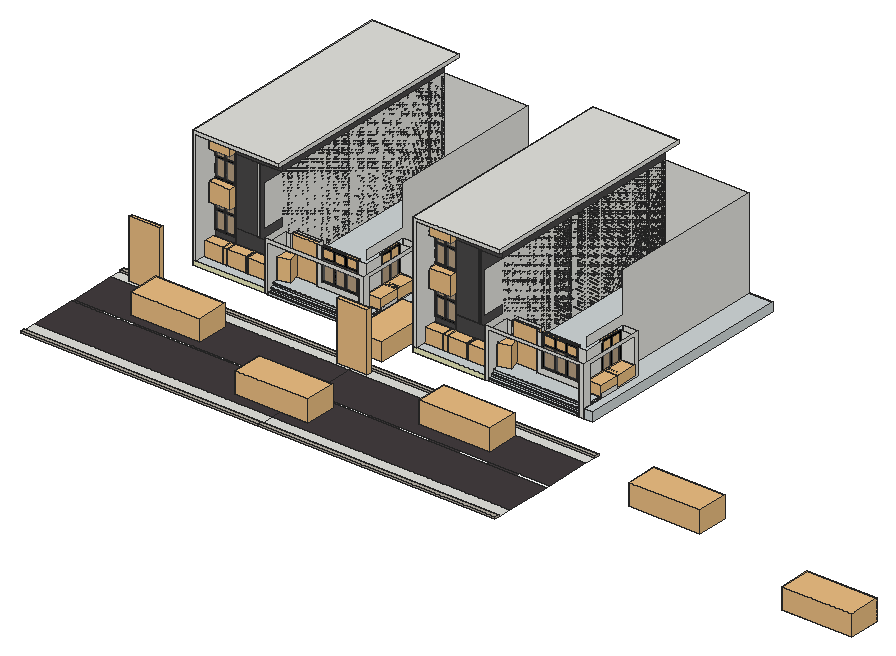
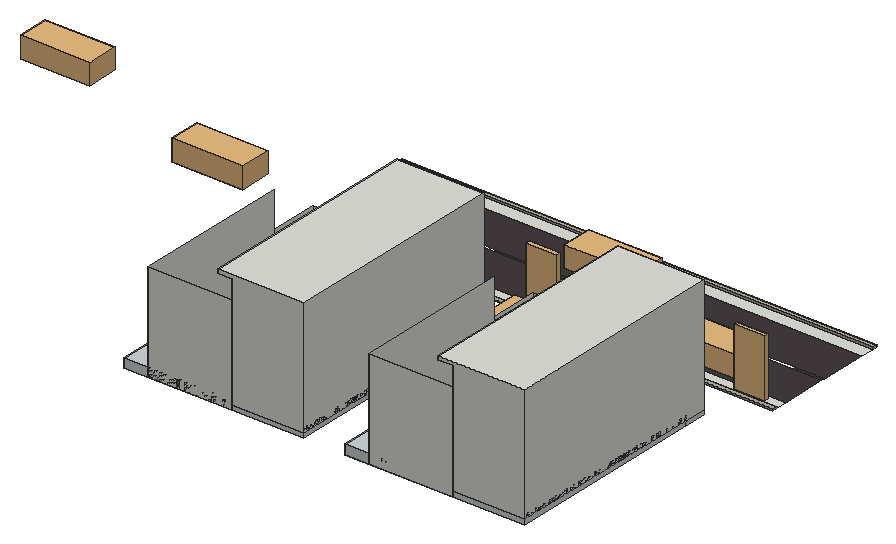
# SketchUp Ruby script. Lengths in inches.
U = 1.inch
M = Sketchup.active_model
def pt(a) = Geom::Point3d.new(a.map { |v| v * U })
def face(e, loops, mat)
  f = e.add_face(loops[0].map { |a| pt(a) })
  loops[1..].each { |l| e.add_face(l.map { |a| pt(a) }).erase! }
  f.material = f.back_material = mat if mat
  f
end
# faces: each face lists its corners as indices into pts; further lists are holes
def faces(e, pts, list, mat = nil) = list.each { |f| face(e, (f[0].is_a?(Array) ? f : [f]).map { |l| l.map { |i| pts[i] } }, mat) }
# xy, xz, yz: faces in a plane at the given z, y or x. An outline is a flat list of corners, or four numbers for a rectangle; further outlines are holes
def ring(l) = l.size == 4 ? [[l[0], l[1]], [l[2], l[1]], [l[2], l[3]], [l[0], l[3]]] : l.each_slice(2).to_a
def flat(e, list, mat, &to3) = list.each { |f| face(e, (f[0].is_a?(Array) ? f : [f]).map { |l| ring(l).map { |u, v| to3.(u, v) } }, mat) }
def xy(e, z, list, mat = nil) = flat(e, list, mat) { |x, y| [x, y, z] }
def xz(e, y, list, mat = nil) = flat(e, list, mat) { |x, z| [x, y, z] }
def yz(e, x, list, mat = nil) = flat(e, list, mat) { |y, z| [x, y, z] }
def lines(e, pts, list) = list.each { |a, b| e.add_line(pt(pts[a]), pt(pts[b])) }
# prism: a flat outline (further loops are holes) pulled along v
def prism(e, loops, v, mat = nil)
  f = face(e, loops, mat); d = Geom::Vector3d.new(v.map { |x| x * U })
  f.pushpull(f.normal.samedirection?(d) ? d.length : -d.length)
end
def box(e, o, s, mat = nil) = prism(e, [[o, [o[0] + s[0], o[1], o[2]], [o[0] + s[0], o[1] + s[1], o[2]], [o[0], o[1] + s[1], o[2]]]], [0, 0, s[2]], mat)
def at(x, y, z, deg = 0) = Geom::Transformation.translation(pt([x, y, z])) * Geom::Transformation.rotation(ORIGIN, Z_AXIS, deg.degrees)
def axes(o, x, y, z) = Geom::Transformation.new([*x, 0, *y, 0, *z, 0, *pt(o).to_a, 1])
def part(name) = M.definitions.add(name)
# library, detail: a bought-in or finely detailed component or shape, given as its bounding box
def library(name, o, s) = part(name).tap { |d| box(d.entities, o, s) }
def detail(e, o, s) = box(e.add_group.entities, o, s)
def put(e, d, t, mat = nil) = e.add_instance(d, t).tap { |i| i.material = mat if mat }
def group(e, t, mat = nil) = e.add_group.tap { |g| g.transformation = t; g.material = mat if mat }.entities
root = M.entities
M.materials.add("1408 AP K082 Hot Ganache-N").color = [74, 72, 72]
M.materials.add("Polycor-Pavers-GEORGIA-MARBLEtm-PEARL-GREY-Tranche-1-4K").color = [207, 214, 215]
M.materials.add("Teddy_Paper").color = [237, 237, 189]
M.materials.add("[Asphalt_New]").color = [67, 60, 62]
M.materials.add("[Color A05]").color = [255, 0, 0]
M.materials.add("[Color M09]").color = [0, 0, 0]
M.materials.add("[Color_000]").color = [255, 255, 255]
M.materials.add("[Stone_Masonry_Multi]").color = [182, 175, 164]
M.materials.add("[Translucent Glass Gray]").color = [128, 128, 128]
M.materials["[Translucent Glass Gray]"].alpha = 0.5
c1 = library("Street Lighting Pole",[31.3125,-4.22,0],[127.34,10.44,259.08])
c2 = library("Group13",[-203.48,36.63,0],[29.68,67.31,50.64])
c3 = library("Group13\#2",[-203.48,36.63,0],[29.68,67.31,50.64])
c4 = part("Group\#61")
p = [[0,1.89,0.38],[0,1.89,1.61],[0,0.72,0],[0,0,0.99],[0,0.72,1.99]]
lines(c4.entities,p,[[0,1],[2,0],[3,2],[4,3],[1,4]])
c5 = part("Component\#76")
p = [[20.45,2.26,80],[20.78,2.41,80]]
lines(c5.entities,p,[[0,1]])
detail(c5.entities,[0,1.93,2.7],[20.05,3.87,77.3])
put(c5.entities,c4,at(9.77,5.02,80,-180))
put(c5.entities,c4,at(11.91,5.02,80,-180))
put(c5.entities,c4,at(13.54,5.02,80,-180))
put(c5.entities,c4,at(7.29,5.02,80,-180))
put(c5.entities,c4,at(6.18,5.02,80,-180))
put(c5.entities,c4,at(8.69,5.02,80,-180))
put(c5.entities,c4,at(17.42,5.04,80,-180))
put(c5.entities,c4,at(18.86,5.04,80,-180))
put(c5.entities,c4,at(15.09,5.02,80,-180))
put(c5.entities,c4,at(16.66,5.04,80,-180))
put(c5.entities,c4,at(2.54,5.02,80,-180))
put(c5.entities,c4,at(1.38,5.02,80,-180))
put(c5.entities,c4,at(4.1,5.02,80,-180))
c6 = library("Group96\#1",[-28.47,-25.5,0],[56.94,51,19.8125])
c7 = library("Group112\#2",[-28.47,-24.66,0],[56.94,49.32,19.8125])
c8 = library("cay+chuoi",[36.12,19.66,0.52],[32.73,35.6,54.38])
c9 = part("weg 1")
xy(c9.entities,0,[[119.79,-0.03,149.12,635.01],[405.36,-0.03,441.44,635.01]])
xy(c9.entities,0,[[149.12,-0.03,272.68,635.01],[272.68,-0.03,280.61,79.35],[280.61,-0.03,405.36,635.01],[272.68,158.73,280.61,238.11],[272.68,317.49,280.61,396.87],
  [272.68,476.25,280.61,555.63]],"[Asphalt_New]")
xy(c9.entities,0,[[272.68,79.35,280.61,158.73],[272.68,238.11,280.61,317.49],[272.68,396.87,280.61,476.25],[272.68,555.63,280.61,635.01]],"[Color_000]")
xy(c9.entities,4.33,[[108.17,0,119.79,635.01]],"[Stone_Masonry_Multi]")
xy(c9.entities,5.12,[[441.44,-0.03,453.25,635.01]],"[Stone_Masonry_Multi]")
xz(c9.entities,-0.03,[[441.44,0,453.25,5.12]],"[Stone_Masonry_Multi]")
xz(c9.entities,0,[[108.17,0,119.79,4.33]],"[Stone_Masonry_Multi]")
xz(c9.entities,635.01,[[108.17,0,119.79,4.33],[441.44,0,453.25,5.12]],"[Stone_Masonry_Multi]")
yz(c9.entities,108.17,[[0,0,635.01,4.33]],"[Stone_Masonry_Multi]")
yz(c9.entities,119.79,[[0,0,635.01,4.33]],"[Stone_Masonry_Multi]")
yz(c9.entities,441.44,[[-0.03,0,635.01,5.12]],"[Stone_Masonry_Multi]")
yz(c9.entities,453.25,[[-0.03,0,635.01,5.12]],"[Stone_Masonry_Multi]")
c10 = part("Group\#1")
xy(c10.entities,-18,[[0,0,192,60],[456.375,0,456.375,60,449.99,60,449.99,7.5,442.99,7.5,442.99,1,200.82,1,200.82,60,0,60,0,600,480,600,480,0]])
xy(c10.entities,-12.875,[[7.5,33,184.5,52.5]])
xy(c10.entities,-12,[[200.82,0,442.99,1]])
xy(c10.entities,-10,[[200.82,0,442.99,8.5]],"Polycor-Pavers-GEORGIA-MARBLEtm-PEARL-GREY-Tranche-1-4K")
xy(c10.entities,-5.0625,[[[0,0,192,60],[7.5,33,184.5,52.5]]])
xy(c10.entities,-4,[[200.82,7.5,442.99,8.5]])
xy(c10.entities,-2,[[200.82,7.5,442.99,16]],"Polycor-Pavers-GEORGIA-MARBLEtm-PEARL-GREY-Tranche-1-4K")
xy(c10.entities,4,[[200.82,15,442.99,16]])
xy(c10.entities,6,[[456.375,0,480,0,480,600,0,600,0,60,200.82,60,200.82,15,442.99,15,442.99,7.5,449.99,7.5,449.99,60,456.375,60]],"Polycor-Pavers-GEORGIA-MARBLEtm-PEARL-GREY-Tranche-1-4K")
xz(c10.entities,0,[[456.375,-18,480,6]])
xz(c10.entities,0,[[200.82,-12,442.99,-10]],"Polycor-Pavers-GEORGIA-MARBLEtm-PEARL-GREY-Tranche-1-4K")
xz(c10.entities,0,[[0,-18,192,-5.0625]],"Teddy_Paper")
xz(c10.entities,1,[[200.82,-18,442.99,-12]],"Polycor-Pavers-GEORGIA-MARBLEtm-PEARL-GREY-Tranche-1-4K")
xz(c10.entities,7.5,[[442.99,-18,449.99,6]])
xz(c10.entities,7.5,[[200.82,-4,442.99,-2]],"Polycor-Pavers-GEORGIA-MARBLEtm-PEARL-GREY-Tranche-1-4K")
xz(c10.entities,8.5,[[200.82,-10,442.99,-4]],"Polycor-Pavers-GEORGIA-MARBLEtm-PEARL-GREY-Tranche-1-4K")
xz(c10.entities,15,[[200.82,4,442.99,6]],"Polycor-Pavers-GEORGIA-MARBLEtm-PEARL-GREY-Tranche-1-4K")
xz(c10.entities,16,[[200.82,-2,442.99,4]],"Polycor-Pavers-GEORGIA-MARBLEtm-PEARL-GREY-Tranche-1-4K")
xz(c10.entities,33,[[7.5,-12.875,184.5,-5.0625]])
xz(c10.entities,52.5,[[7.5,-12.875,184.5,-5.0625]])
xz(c10.entities,60,[[0,-18,192,-5.0625],[192,-18,200.82,6],[449.99,-18,456.375,6],[0,-5.0625,192,6]])
xz(c10.entities,600,[[0,-18,480,6]])
yz(c10.entities,0,[[0,-18,60,-5.0625],[60,-18,600,6]])
yz(c10.entities,7.5,[[33,-12.875,52.5,-5.0625]])
yz(c10.entities,184.5,[[33,-12.875,52.5,-5.0625]])
yz(c10.entities,192,[[0,-18,60,-5.0625]])
yz(c10.entities,200.82,[[1,-18,1,-12,0,-12,0,-10,8.5,-10,8.5,-4,7.5,-4,7.5,-2,16,-2,16,4,15,4,15,6,60,6,60,-18]])
yz(c10.entities,442.99,[[1,-18,7.5,-18,7.5,-10,0,-10,0,-12,1,-12],[7.5,-10,8.5,-4],[7.5,-2,7.5,6,15,6,15,4,16,4,16,-2]])
yz(c10.entities,449.99,[[7.5,-18,60,6]])
yz(c10.entities,456.375,[[0,-18,60,6]])
yz(c10.entities,480,[[0,-18,600,6]])
c11 = library("Component",[-22.57,36.53,5.61],[7.19,69.19,99.57])
c12 = library("curtain",[-132.09,64.9,20.5],[94.35,4.27,84.68])
c13 = library("Group8",[-183.25,9.15,0],[25.91,56.79,43.93])
c14 = library("Untitled\#1",[-3930.05,580.88,0.02],[81.53,169.31,48.44])
c15 = library("bmw m6",[0,0,0],[74.56,175.18,49.66])
c16 = library("araç",[-7.9,-14.14,0],[84.07,190.26,56.29])
c17 = library("MERCEDES LIGHT",[-74.97,-97.73,0.18],[82.22,195.9,56.22])
c18 = part("cars")
put(c18.entities,c15,axes([-854.13,88.1875,0],[0,1.12,0],[-1.05539,0,0],[0,0,1.12246]))
put(c18.entities,c16,at(-104.32,108.73,0,90))
put(c18.entities,c17,at(-555.31,27.51,5.12,90))
put(c18.entities,c16,at(456.62,108.73,0,90))
put(c18.entities,c15,axes([807.37,-43.625,0],[0,1.12,0],[1.05539,0,0],[0,0,1.12246]))
xy(root,-4.3125,[[293.22,449.7,293.22,1049.7,518.04,1049.7,518.04,629.7,557.59,629.7,557.59,449.7,551.21,449.7,551.21,509.7,384.73,509.7,384.73,530.01,315.54,530.01,315.54,509.7,302.04,509.7,302.04,449.7],[544.21,449.7,551.21,457.2],[883.03,449.7,883.03,1049.7,1107.85,1049.7,1107.85,629.7,1147.4,629.7,1147.4,449.7,1141.02,449.7,1141.02,509.7,974.54,509.7,974.54,530.01,905.35,530.01,905.35,509.7,891.85,509.7,891.85,449.7],[1134.02,449.7,1141.02,457.2]])
xy(root,19.6875,[[551.21,468.65,557.59,509.7],[1141.02,468.65,1147.4,509.7]])
xy(root,22.13,[[522.83,514.49,552.8,616.09],[1112.64,514.49,1142.62,616.09]])
xy(root,28.51,[[[518.04,509.7,557.59,620.88],[522.83,514.49,552.8,616.09]],[[1107.85,509.7,1147.4,620.88],[1112.64,514.49,1142.62,616.09]]])
xy(root,34.1875,[[398.04,512.7,430.93,533.7],[430.93,512.7,461.15,533.7],[461.15,512.7,494.04,533.7],[987.85,512.7,1020.74,533.7],[1020.74,512.7,1050.96,533.7],
  [1050.96,512.7,1083.85,533.7]])
xy(root,34.1875,[[398.04,509.7,494.04,512.7],[987.85,509.7,1083.85,512.7],[516.04,559.44,518.04,590.16],[1105.85,559.44,1107.85,590.16],[516.04,590.16,518.04,620.88],
  [1105.85,590.16,1107.85,620.88]],"[Color M09]")
xy(root,34.86,[[501.6,560.12,516.04,591.16],[1091.41,560.12,1105.85,591.16],[501.6,591.16,516.04,620.2],[1091.41,591.16,1105.85,620.2]])
xy(root,36.86,[[400.71,509.7,430.93,511.2],[433.56,509.7,461.15,511.2],[463.98,509.7,491.36,511.2],[990.53,509.7,1020.74,511.2],[1023.37,509.7,1050.96,511.2],
  [1053.79,509.7,1081.17,511.2],[400.71,511.2,430.93,512.7],[433.56,511.2,461.15,512.7],[463.98,511.2,491.36,512.7],[990.53,511.2,1020.74,512.7],
  [1023.37,511.2,1050.96,512.7],[1053.79,511.2,1081.17,512.7],[516.04,562.12,517.04,589.16],[517.04,562.12,518.04,589.16],[1105.85,562.12,1106.85,589.16],
  [1106.85,562.12,1107.85,589.16],[516.04,589.16,518.04,590.16],[1105.85,589.16,1107.85,590.16],[516.04,590.16,518.04,591.16],[1105.85,590.16,1107.85,591.16],
  [516.04,591.16,517.04,618.2],[517.04,591.16,518.04,618.2],[1105.85,591.16,1106.85,618.2],[1106.85,591.16,1107.85,618.2]],"[Color M09]")
xz(root,449.7,[[293.22,-4.3125,302.04,-4.3125,302.04,118.87,544.21,118.87,544.21,-4.3125,557.59,-4.3125,557.59,127.6875,293.22,127.6875],[883.03,-4.3125,891.85,-4.3125,891.85,118.87,1134.02,118.87,1134.02,-4.3125,1147.4,-4.3125,1147.4,127.6875,883.03,127.6875]])
xz(root,457.2,[[544.21,-4.3125,551.21,118.87],[1134.02,-4.3125,1141.02,118.87]])
xz(root,468.65,[[551.21,19.6875,557.59,118.87],[1141.02,19.6875,1147.4,118.87]])
xz(root,509.7,[[302.04,-4.3125,315.54,118.87],[384.73,-4.3125,551.21,-4.3125,551.21,28.51,518.04,28.51,518.04,118.87,494.04,118.87,494.04,34.1875,398.04,34.1875,398.04,118.87,384.73,118.87],[891.85,-4.3125,905.35,118.87],[974.54,-4.3125,1141.02,-4.3125,1141.02,28.51,1107.85,28.51,1107.85,118.87,1083.85,118.87,1083.85,34.1875,987.85,34.1875,987.85,118.87,974.54,118.87],[551.21,19.6875,557.59,28.51],
  [1141.02,19.6875,1147.4,28.51]])
xz(root,509.7,[[[398.04,34.1875,494.04,118.87],[400.71,36.86,430.93,89.9],[433.56,36.86,461.15,89.9],[463.98,36.86,491.36,89.9],[400.71,92.58,430.93,116.1875],[433.56,92.58,461.15,116.1875],[463.98,92.58,491.36,116.1875]],[[987.85,34.1875,1083.85,118.87],[990.53,36.86,1020.74,89.9],[1023.37,36.86,1050.96,89.9],[1053.79,36.86,1081.17,89.9],[990.53,92.58,1020.74,116.1875],[1023.37,92.58,1050.96,116.1875],[1053.79,92.58,1081.17,116.1875]]],"[Color M09]")
xz(root,511.2,[[400.71,36.86,430.93,89.9],[433.56,36.86,461.15,89.9],[463.98,36.86,491.36,89.9],[990.53,36.86,1020.74,89.9],[1023.37,36.86,1050.96,89.9],
  [1053.79,36.86,1081.17,89.9]],"[Translucent Glass Gray]")
xz(root,512.7,[[430.93,34.1875,433.56,89.9],[1020.74,34.1875,1023.37,89.9]])
xz(root,512.7,[[398.04,34.1875,430.93,36.86],[433.56,34.1875,461.15,36.86],[461.15,34.1875,463.98,89.9],[463.98,34.1875,491.36,36.86],[491.36,34.1875,494.04,89.9],
  [987.85,34.1875,1020.74,36.86],[1023.37,34.1875,1050.96,36.86],[1050.96,34.1875,1053.79,89.9],[1053.79,34.1875,1081.17,36.86],[1081.17,34.1875,1083.85,89.9],
  [398.04,36.86,400.71,89.9],[987.85,36.86,990.53,89.9]],"[Color M09]")
xz(root,514.49,[[522.83,22.13,551.21,28.51],[551.21,22.13,552.8,28.51],[1112.64,22.13,1141.02,28.51],[1141.02,22.13,1142.62,28.51]])
xz(root,530.01,[[315.54,-4.3125,384.73,118.87],[905.35,-4.3125,974.54,118.87]])
xz(root,533.7,[[398.04,34.1875,430.93,89.9],[430.93,34.1875,461.15,89.9],[461.15,34.1875,494.04,89.9],[987.85,34.1875,1020.74,89.9],[1020.74,34.1875,1050.96,89.9],
  [1050.96,34.1875,1083.85,89.9]])
xz(root,559.44,[[516.04,34.1875,518.04,118.87],[1105.85,34.1875,1107.85,118.87]],"[Color M09]")
xz(root,560.12,[[501.6,34.86,516.04,89.9],[1091.41,34.86,1105.85,89.9]])
xz(root,561.12,[[516.04,36.86,518.04,89.9],[1105.85,36.86,1107.85,89.9]])
xz(root,562.12,[[516.04,36.86,517.04,89.9],[517.04,36.86,518.04,89.9],[1105.85,36.86,1106.85,89.9],[1106.85,36.86,1107.85,89.9]],"[Color M09]")
xz(root,589.16,[[516.04,36.86,517.04,89.9],[517.04,36.86,518.04,89.9],[1105.85,36.86,1106.85,89.9],[1106.85,36.86,1107.85,89.9]],"[Color M09]")
xz(root,590.16,[[516.04,34.1875,518.04,36.86],[1105.85,34.1875,1107.85,36.86]],"[Color M09]")
xz(root,591.16,[[516.04,36.86,517.04,89.9],[517.04,36.86,518.04,89.9],[1105.85,36.86,1106.85,89.9],[1106.85,36.86,1107.85,89.9]],"[Color M09]")
xz(root,616.09,[[522.83,22.13,552.8,28.51],[1112.64,22.13,1142.62,28.51]])
xz(root,618.2,[[516.04,36.86,517.04,89.9],[517.04,36.86,518.04,89.9],[1105.85,36.86,1106.85,89.9],[1106.85,36.86,1107.85,89.9]],"[Color M09]")
xz(root,620.2,[[501.6,34.86,516.04,89.9],[1091.41,34.86,1105.85,89.9]])
xz(root,620.88,[[518.04,28.51,557.59,118.87],[1107.85,28.51,1147.4,118.87]])
xz(root,620.88,[[516.04,34.1875,518.04,118.87],[1105.85,34.1875,1107.85,118.87]],"[Color M09]")
xz(root,629.7,[[518.04,-4.3125,557.59,127.6875],[1107.85,-4.3125,1147.4,127.6875]])
xz(root,1049.7,[[293.22,-4.3125,518.04,259.6875],[883.03,-4.3125,1107.85,259.6875]])
yz(root,293.22,[[449.7,-4.3125,449.7,127.6875,509.7,127.6875,509.7,151.6875,449.7,151.6875,449.7,259.6875,1049.7,259.6875,1049.7,-4.3125]])
yz(root,302.04,[[449.7,-4.3125,509.7,118.87]])
yz(root,315.54,[[509.7,-4.3125,530.01,118.87]])
yz(root,384.73,[[509.7,-4.3125,530.01,118.87]])
yz(root,398.04,[[512.7,34.1875,533.7,89.9]])
yz(root,398.04,[[509.7,34.1875,512.7,118.87]],"[Color M09]")
yz(root,400.71,[[509.7,36.86,511.2,89.9],[511.2,36.86,512.7,89.9]],"[Color M09]")
yz(root,430.93,[[509.7,36.86,511.2,89.9],[511.2,36.86,512.7,89.9]],"[Color M09]")
yz(root,433.56,[[509.7,36.86,511.2,89.9],[511.2,36.86,512.7,89.9]],"[Color M09]")
yz(root,461.15,[[509.7,36.86,511.2,89.9],[511.2,36.86,512.7,89.9]],"[Color M09]")
yz(root,463.98,[[509.7,36.86,511.2,89.9],[511.2,36.86,512.7,89.9]],"[Color M09]")
yz(root,491.36,[[509.7,36.86,511.2,89.9],[511.2,36.86,512.7,89.9]],"[Color M09]")
yz(root,494.04,[[512.7,34.1875,533.7,89.9]])
yz(root,494.04,[[509.7,34.1875,512.7,118.87]],"[Color M09]")
yz(root,501.6,[[560.12,34.86,591.16,89.9],[591.16,34.86,620.2,89.9]])
yz(root,516.04,[[562.12,34.86,589.16,36.86]])
yz(root,516.04,[[[559.44,34.1875,620.88,118.87],[560.12,34.86,620.2,118.1875]],[560.12,34.86,562.12,89.9],[589.16,34.86,590.16,36.86],[590.16,34.86,591.16,36.86],[591.16,34.86,618.2,36.86],
  [618.2,34.86,620.2,89.9],[589.16,36.86,591.16,89.9]],"[Color M09]")
yz(root,517.04,[[562.12,36.86,589.16,89.9],[591.16,36.86,618.2,89.9]],"[Translucent Glass Gray]")
yz(root,518.04,[[629.7,-4.3125,1049.7,-4.3125,1049.7,259.6875,629.7,259.6875,629.7,151.6875,509.7,151.6875,509.7,127.6875,629.7,127.6875],[509.7,28.51,620.88,28.51,620.88,34.1875,559.44,34.1875,559.44,118.87,509.7,118.87]])
yz(root,518.04,[[[559.44,34.1875,590.16,34.1875,590.16,36.86,562.12,36.86,562.12,89.9,589.16,89.9,589.16,36.86,591.16,36.86,591.16,89.9,618.2,89.9,618.2,36.86,590.16,36.86,590.16,34.1875,620.88,34.1875,620.88,118.87,559.44,118.87],[591.16,92.58,618.2,116.1875],[562.12,92.58,589.16,116.1875]]],"[Color M09]")
yz(root,522.83,[[514.49,22.13,616.09,28.51]])
yz(root,544.21,[[449.7,-4.3125,457.2,118.87]])
yz(root,551.21,[[457.2,-4.3125,457.2,118.87,468.65,118.87,468.65,19.6875,509.7,19.6875,509.7,-4.3125]])
yz(root,552.8,[[514.49,22.13,616.09,28.51]])
yz(root,557.59,[[[449.7,-4.3125,629.7,127.6875],[468.65,19.6875,468.65,118.87,620.88,118.87,620.88,28.51,509.7,28.51,509.7,19.6875]]])
yz(root,883.03,[[449.7,-4.3125,449.7,127.6875,509.7,127.6875,509.7,151.6875,449.7,151.6875,449.7,259.6875,1049.7,259.6875,1049.7,-4.3125]])
yz(root,891.85,[[449.7,-4.3125,509.7,118.87]])
yz(root,905.35,[[509.7,-4.3125,530.01,118.87]])
yz(root,974.54,[[509.7,-4.3125,530.01,118.87]])
yz(root,987.85,[[512.7,34.1875,533.7,89.9]])
yz(root,987.85,[[509.7,34.1875,512.7,118.87]],"[Color M09]")
yz(root,990.53,[[509.7,36.86,511.2,89.9],[511.2,36.86,512.7,89.9]],"[Color M09]")
yz(root,1020.74,[[509.7,36.86,511.2,89.9],[511.2,36.86,512.7,89.9]],"[Color M09]")
yz(root,1023.37,[[509.7,36.86,511.2,89.9],[511.2,36.86,512.7,89.9]],"[Color M09]")
yz(root,1050.96,[[509.7,36.86,511.2,89.9],[511.2,36.86,512.7,89.9]],"[Color M09]")
yz(root,1053.79,[[509.7,36.86,511.2,89.9],[511.2,36.86,512.7,89.9]],"[Color M09]")
yz(root,1081.17,[[509.7,36.86,511.2,89.9],[511.2,36.86,512.7,89.9]],"[Color M09]")
yz(root,1083.85,[[512.7,34.1875,533.7,89.9]])
yz(root,1083.85,[[509.7,34.1875,512.7,118.87]],"[Color M09]")
yz(root,1091.41,[[560.12,34.86,591.16,89.9],[591.16,34.86,620.2,89.9]])
yz(root,1105.85,[[562.12,34.86,589.16,36.86]])
yz(root,1105.85,[[[559.44,34.1875,620.88,118.87],[560.12,34.86,620.2,118.1875]],[560.12,34.86,562.12,89.9],[589.16,34.86,590.16,36.86],[590.16,34.86,591.16,36.86],[591.16,34.86,618.2,36.86],
  [618.2,34.86,620.2,89.9],[589.16,36.86,591.16,89.9]],"[Color M09]")
yz(root,1106.85,[[562.12,36.86,589.16,89.9],[591.16,36.86,618.2,89.9]],"[Translucent Glass Gray]")
yz(root,1107.85,[[629.7,-4.3125,1049.7,-4.3125,1049.7,259.6875,629.7,259.6875,629.7,151.6875,509.7,151.6875,509.7,127.6875,629.7,127.6875],[509.7,28.51,620.88,28.51,620.88,34.1875,559.44,34.1875,559.44,118.87,509.7,118.87]])
yz(root,1107.85,[[[559.44,34.1875,590.16,34.1875,590.16,36.86,562.12,36.86,562.12,89.9,589.16,89.9,589.16,36.86,591.16,36.86,591.16,89.9,618.2,89.9,618.2,36.86,590.16,36.86,590.16,34.1875,620.88,34.1875,620.88,118.87,559.44,118.87],[591.16,92.58,618.2,116.1875],[562.12,92.58,589.16,116.1875]]],"[Color M09]")
yz(root,1112.64,[[514.49,22.13,616.09,28.51]])
yz(root,1134.02,[[449.7,-4.3125,457.2,118.87]])
yz(root,1141.02,[[457.2,-4.3125,457.2,118.87,468.65,118.87,468.65,19.6875,509.7,19.6875,509.7,-4.3125]])
yz(root,1142.62,[[514.49,22.13,616.09,28.51]])
yz(root,1147.4,[[[449.7,-4.3125,629.7,127.6875],[468.65,19.6875,468.65,118.87,620.88,118.87,620.88,28.51,509.7,28.51,509.7,19.6875]]])
put(root,c1,axes([141.65,319.78,-4.3125],[-0.6408,0,0],[0,-1,0],[0,0,0.6]))
put(root,c2,at(66.93,302.57,-3.77,-90))
put(root,c3,at(122.68,302.57,-3.77,-90))
g1 = group(root,at(101.22,509.7,19.6875))
xy(g1,-11.0625,[[0,-60,0,540,192,540,192,0,65.94,0,65.94,2,9,2,9,-60]])
xy(g1,36.75,[[9,2,65.94,5],[35.97,5,65.94,22.6875]])
xy(g1,39.75,[[8.8125,5,35.78,22.6875],[35.78,5,35.97,22.6875]])
xy(g1,39.75,[[12,2,35.97,3.5],[38.97,2,62.94,3.5],[12,3.5,35.97,5],[38.97,3.5,62.94,5]],"[Color M09]")
xy(g1,62.03,[[65.94,0,125.97,2],[125.97,0,131.97,2],[131.97,0,192,2],[65.94,5,66.13,22.6875]])
xy(g1,62.31,[[65.94,0,125.97,2],[131.97,0,192,2]])
xy(g1,85.86,[[8.8125,5,9,22.6875]])
xy(g1,86.04,[[65.94,5,66.13,22.6875]])
xy(g1,86.04,[[12,2,35.97,3.5],[38.97,2,62.94,3.5],[12,3.5,35.97,5],[38.97,3.5,62.94,5]],"[Color M09]")
xy(g1,89.04,[[12,2,35.97,3.5],[38.97,2,62.94,3.5],[12,3.5,35.97,5],[38.97,3.5,62.94,5]],"[Color M09]")
xy(g1,109.875,[[35.97,2,38.97,5]])
xy(g1,109.875,[[12,2,35.97,3.5],[38.97,2,62.94,3.5],[12,3.5,35.97,5],[38.97,3.5,62.94,5]],"[Color M09]")
xy(g1,112.875,[[9,2,65.94,5],[35.97,5,65.94,22.6875]])
xy(g1,113.0625,[[9,5,35.78,22.6875]])
xy(g1,162.1875,[[9,2,65.94,5],[9,5,38.97,22.6875],[38.97,5,65.94,22.6875]])
xy(g1,165.375,[[12,2,35.97,3.5],[38.97,2,62.94,3.5],[12,3.5,35.97,5],[38.97,3.5,62.94,5]],"[Color M09]")
xy(g1,212.9,[[12,2,35.97,3.5],[38.97,2,62.94,3.5],[12,3.5,35.97,5],[38.97,3.5,62.94,5]],"[Color M09]")
xy(g1,215.9,[[12,2,35.97,5],[38.97,2,62.94,3.5],[38.97,3.5,62.94,5]],"[Color M09]")
xy(g1,237,[[12,2,35.97,3.5],[38.97,2,62.94,3.5],[12,3.5,35.97,5],[38.97,3.5,62.94,5]],"[Color M09]")
xy(g1,239.72,[[65.94,0,125.97,2],[131.97,0,192,2]])
xy(g1,240,[[65.94,0,125.97,2],[125.97,0,131.97,2],[131.97,0,192,2],[9,2,65.94,5],[9,5,35.97,22.6875],
  [35.97,5,65.94,22.6875]])
xy(g1,291,[[9,-60,9,2,65.94,2,65.94,0,192,0,192,540,230.1875,540,230.1875,-60]])
xy(g1,300,[[0,-60,230.1875,540]])
xz(g1,-60,[[0,-11.0625,9,-11.0625,9,291,230.1875,291,230.1875,300,0,300]])
xz(g1,0,[[65.94,-11.0625,192,62.03],[65.94,62.31,125.97,239.72],[131.97,62.31,192,239.72],[65.94,240,192,291]],"1408 AP K082 Hot Ganache-N")
xz(g1,2,[[65.94,62.03,125.97,62.31],[125.97,62.03,131.97,240],[131.97,62.03,192,62.31],[65.94,62.31,125.97,239.72],[65.94,239.72,125.97,240],
  [131.97,239.72,192,240]])
xz(g1,2,[[9,-11.0625,65.94,36.75]],"1408 AP K082 Hot Ganache-N")
xz(g1,2,[[[9,36.75,65.94,112.875],[12,39.75,35.97,86.04],[38.97,39.75,62.94,86.04],[12,89.04,12,109.875,62.94,109.875,62.94,89.04,38.97,89.04,38.97,109.875,35.97,109.875,35.97,89.04]],[[9,162.1875,65.94,240],[12,165.375,35.97,212.9],[38.97,165.375,62.94,212.9],[38.97,215.9,62.94,237],[12,215.9,35.97,237]]],"[Color M09]")
xz(g1,3.5,[[12,39.75,35.97,86.04],[38.97,39.75,62.94,86.04],[12,89.04,35.97,109.875],[38.97,89.04,62.94,109.875],[12,165.375,35.97,212.9],
  [38.97,165.375,62.94,212.9],[12,215.4,36.54,237],[38.97,215.9,62.94,237]],"[Translucent Glass Gray]")
xz(g1,5,[[9,36.75,35.97,39.75],[35.97,36.75,38.97,86.04],[38.97,36.75,65.94,39.75],[8.8125,39.75,9,85.86],[9,39.75,12,85.86],
  [35.78,39.75,35.97,86.04],[62.94,39.75,65.94,62.03],[62.94,62.03,65.94,62.31],[65.94,62.03,66.13,62.31],[62.94,62.31,65.94,86.04],
  [65.94,62.31,66.13,86.04],[9,85.86,12,86.04],[12,85.86,35.78,86.04],[9,86.04,35.78,89.04],[35.78,86.04,38.97,86.04,38.97,109.875,35.97,109.875,35.97,89.04,35.78,89.04],
  [38.97,86.04,65.94,89.04],[9,89.04,12,89.23],[12,89.04,35.78,89.23],[35.78,89.04,35.97,109.875],[62.94,89.04,65.94,112.875],
  [9,89.23,12,109.875],[9,109.875,35.78,112.875],[35.78,109.875,35.97,112.875],[35.97,109.875,38.97,112.875],[38.97,109.875,62.94,112.875],
  [9,112.875,35.78,113.0625],[9,162.1875,35.97,165.375],[35.97,162.1875,38.97,212.9],[38.97,162.1875,65.94,165.375],[9,165.375,12,212.9],
  [62.94,165.375,65.94,212.9],[9,212.9,35.97,215.9],[35.97,212.9,38.97,240],[38.97,212.9,65.94,215.9],[9,215.9,12,240],
  [62.94,215.9,65.94,237],[12,237,35.97,240],[38.97,237,65.94,240]])
xz(g1,22.6875,[[35.97,36.75,65.94,36.75,65.94,62.03,66.13,62.03,66.13,86.04,35.97,86.04],[8.8125,39.75,35.78,85.86],[35.78,39.75,35.97,86.04],[9,85.86,35.78,89.23],[35.78,86.04,65.94,86.04,65.94,112.875,35.97,112.875,35.97,89.04,35.78,89.04],
  [35.78,89.04,35.97,109.875],[9,89.23,35.78,113.0625],[9,162.1875,38.97,212.9],[38.97,162.1875,65.94,212.9],[9,212.9,35.97,240],
  [35.97,212.9,65.94,240]])
xz(g1,540,[[0,-11.0625,0,300,230.1875,300,230.1875,291,192,291,192,-11.0625]])
yz(g1,0,[[-60,-11.0625,540,300]])
yz(g1,8.8125,[[5,39.75,22.6875,85.86]])
yz(g1,9,[[-60,-11.0625,2,291],[2,36.75,5,112.875],[5,85.86,22.6875,89.23],[5,89.23,22.6875,113.0625],[2,162.1875,5,240],
  [5,162.1875,22.6875,212.9],[5,212.9,22.6875,240]])
yz(g1,12,[[2,39.75,3.5,86.04],[3.5,39.75,5,86.04],[2,89.04,3.5,109.875],[3.5,89.04,5,109.875],[2,165.375,3.5,212.9],
  [3.5,165.375,5,212.9],[2,215.9,3.5,237],[3.5,215.9,5,237]],"[Color M09]")
yz(g1,35.97,[[5,36.75,22.6875,39.75]])
yz(g1,35.97,[[2,39.75,3.5,86.04],[3.5,39.75,5,86.04],[2,89.04,3.5,109.875],[3.5,89.04,5,109.875],[2,165.375,3.5,212.9],
  [3.5,165.375,5,212.9],[2,215.9,5,237]],"[Color M09]")
yz(g1,38.97,[[2,39.75,3.5,86.04],[3.5,39.75,5,86.04],[2,89.04,3.5,109.875],[3.5,89.04,5,109.875],[2,165.375,3.5,212.9],
  [3.5,165.375,5,212.9],[2,215.9,3.5,237],[3.5,215.9,5,237]],"[Color M09]")
yz(g1,62.94,[[2,39.75,3.5,62.03],[3.5,39.75,5,62.03],[2,62.03,3.5,62.31],[3.5,62.03,5,62.31]])
yz(g1,62.94,[[2,62.31,3.5,86.04],[3.5,62.31,5,86.04],[2,89.04,3.5,109.875],[3.5,89.04,5,109.875],[2,165.375,3.5,212.9],
  [3.5,165.375,5,212.9],[2,215.9,3.5,237],[3.5,215.9,5,237]],"[Color M09]")
yz(g1,65.94,[[0,-11.0625,2,62.03],[2,36.75,5,62.03],[5,36.75,22.6875,62.03],[2,62.03,5,62.31],[0,62.31,2,239.72],
  [2,62.31,5,112.875],[5,86.04,22.6875,112.875],[2,162.1875,5,239.72],[5,162.1875,22.6875,212.9],[5,212.9,22.6875,240],
  [2,239.72,5,240],[0,240,2,291]])
yz(g1,66.13,[[5,62.03,22.6875,62.31],[5,62.31,22.6875,86.04]])
yz(g1,125.97,[[0,62.31,2,239.72]])
yz(g1,131.97,[[0,62.31,2,239.72]])
yz(g1,192,[[0,-11.0625,540,-11.0625,540,291,0,291,0,240,2,240,2,239.72,0,239.72,0,62.31,2,62.31,2,62.03,0,62.03]],"1408 AP K082 Hot Ganache-N")
yz(g1,230.1875,[[-60,291,540,300]])
put(g1,c5,axes([61.93,4.77,37.34],[-2.59641,0,0],[0,0.684,0],[0,0,0.92358]))
put(g1,c5,axes([61.93,4.77,163.7],[-2.59641,0,0],[0,0.684,0],[0,0,0.92358]))
put(g1,c6,axes([37.47,2,265.5],[1,0,0],[0,0,1],[0,-1,0]))
put(g1,c7,axes([37.47,2,137.53],[1,0,0],[0,0,1],[0,-1,0]))
put(root,c3,at(185.24,302.57,-3.77,-90))
put(root,c8,at(272.97,449.07,19.875,15))
put(root,c9,at(0.03,453.25,-4.3125,-90))
put(root,c10,at(101.22,449.7,13.6875),"Polycor-Pavers-GEORGIA-MARBLEtm-PEARL-GREY-Tranche-1-4K")
put(root,c11,at(279,498.54,13.6875,-90))
put(root,c12,at(530.13,449.7,13.6875))
put(root,c12,axes([580.89,641.46,13.01],[0,0.61,0],[-1,0,0],[0,0,1]))
put(root,c13,axes([773.98,497.25,22.13],[1.38,0,0],[0,1.17,0],[0,0,0.61]))
put(root,c13,axes([779.23,554.02,22.13],[1.40866,0,0],[0,1,0],[0,0,0.61]))
put(root,c14,at(4520.13,-211.18,0))
put(root,c1,axes([696.84,319.78,-4.3125],[-0.6408,0,0],[0,-1,0],[0,0,0.6]))
put(root,c2,at(656.74,302.57,-3.77,-90))
put(root,c3,at(712.49,302.57,-3.77,-90))
g2 = group(root,at(691.03,509.7,19.6875))
xy(g2,-11.0625,[[0,-60,0,540,192,540,192,0,65.94,0,65.94,2,9,2,9,-60]])
xy(g2,36.75,[[9,2,65.94,5],[35.97,5,65.94,22.6875]])
xy(g2,39.75,[[8.8125,5,35.78,22.6875],[35.78,5,35.97,22.6875]])
xy(g2,39.75,[[12,2,35.97,3.5],[38.97,2,62.94,3.5],[12,3.5,35.97,5],[38.97,3.5,62.94,5]],"[Color M09]")
xy(g2,62.03,[[65.94,0,125.97,2],[125.97,0,131.97,2],[131.97,0,192,2],[65.94,5,66.13,22.6875]])
xy(g2,62.31,[[65.94,0,125.97,2],[131.97,0,192,2]])
xy(g2,85.86,[[8.8125,5,9,22.6875]])
xy(g2,86.04,[[65.94,5,66.13,22.6875]])
xy(g2,86.04,[[12,2,35.97,3.5],[38.97,2,62.94,3.5],[12,3.5,35.97,5],[38.97,3.5,62.94,5]],"[Color M09]")
xy(g2,89.04,[[12,2,35.97,3.5],[38.97,2,62.94,3.5],[12,3.5,35.97,5],[38.97,3.5,62.94,5]],"[Color M09]")
xy(g2,109.875,[[35.97,2,38.97,5]])
xy(g2,109.875,[[12,2,35.97,3.5],[38.97,2,62.94,3.5],[12,3.5,35.97,5],[38.97,3.5,62.94,5]],"[Color M09]")
xy(g2,112.875,[[9,2,65.94,5],[35.97,5,65.94,22.6875]])
xy(g2,113.0625,[[9,5,35.78,22.6875]])
xy(g2,162.1875,[[9,2,65.94,5],[9,5,38.97,22.6875],[38.97,5,65.94,22.6875]])
xy(g2,165.375,[[12,2,35.97,3.5],[38.97,2,62.94,3.5],[12,3.5,35.97,5],[38.97,3.5,62.94,5]],"[Color M09]")
xy(g2,212.9,[[12,2,35.97,3.5],[38.97,2,62.94,3.5],[12,3.5,35.97,5],[38.97,3.5,62.94,5]],"[Color M09]")
xy(g2,215.9,[[12,2,35.97,5],[38.97,2,62.94,3.5],[38.97,3.5,62.94,5]],"[Color M09]")
xy(g2,237,[[12,2,35.97,3.5],[38.97,2,62.94,3.5],[12,3.5,35.97,5],[38.97,3.5,62.94,5]],"[Color M09]")
xy(g2,239.72,[[65.94,0,125.97,2],[131.97,0,192,2]])
xy(g2,240,[[65.94,0,125.97,2],[125.97,0,131.97,2],[131.97,0,192,2],[9,2,65.94,5],[9,5,35.97,22.6875],
  [35.97,5,65.94,22.6875]])
xy(g2,291,[[9,-60,9,2,65.94,2,65.94,0,192,0,192,540,230.1875,540,230.1875,-60]])
xy(g2,300,[[0,-60,230.1875,540]])
xz(g2,-60,[[0,-11.0625,9,-11.0625,9,291,230.1875,291,230.1875,300,0,300]])
xz(g2,0,[[65.94,-11.0625,192,62.03],[65.94,62.31,125.97,239.72],[131.97,62.31,192,239.72],[65.94,240,192,291]],"1408 AP K082 Hot Ganache-N")
xz(g2,2,[[65.94,62.03,125.97,62.31],[125.97,62.03,131.97,240],[131.97,62.03,192,62.31],[65.94,62.31,125.97,239.72],[65.94,239.72,125.97,240],
  [131.97,239.72,192,240]])
xz(g2,2,[[9,-11.0625,65.94,36.75]],"1408 AP K082 Hot Ganache-N")
xz(g2,2,[[[9,36.75,65.94,112.875],[12,39.75,35.97,86.04],[38.97,39.75,62.94,86.04],[12,89.04,12,109.875,62.94,109.875,62.94,89.04,38.97,89.04,38.97,109.875,35.97,109.875,35.97,89.04]],[[9,162.1875,65.94,240],[12,165.375,35.97,212.9],[38.97,165.375,62.94,212.9],[38.97,215.9,62.94,237],[12,215.9,35.97,237]]],"[Color M09]")
xz(g2,3.5,[[12,39.75,35.97,86.04],[38.97,39.75,62.94,86.04],[12,89.04,35.97,109.875],[38.97,89.04,62.94,109.875],[12,165.375,35.97,212.9],
  [38.97,165.375,62.94,212.9],[12,215.4,36.54,237],[38.97,215.9,62.94,237]],"[Translucent Glass Gray]")
xz(g2,5,[[9,36.75,35.97,39.75],[35.97,36.75,38.97,86.04],[38.97,36.75,65.94,39.75],[8.8125,39.75,9,85.86],[9,39.75,12,85.86],
  [35.78,39.75,35.97,86.04],[62.94,39.75,65.94,62.03],[62.94,62.03,65.94,62.31],[65.94,62.03,66.13,62.31],[62.94,62.31,65.94,86.04],
  [65.94,62.31,66.13,86.04],[9,85.86,12,86.04],[12,85.86,35.78,86.04],[9,86.04,35.78,89.04],[35.78,86.04,38.97,86.04,38.97,109.875,35.97,109.875,35.97,89.04,35.78,89.04],
  [38.97,86.04,65.94,89.04],[9,89.04,12,89.23],[12,89.04,35.78,89.23],[35.78,89.04,35.97,109.875],[62.94,89.04,65.94,112.875],
  [9,89.23,12,109.875],[9,109.875,35.78,112.875],[35.78,109.875,35.97,112.875],[35.97,109.875,38.97,112.875],[38.97,109.875,62.94,112.875],
  [9,112.875,35.78,113.0625],[9,162.1875,35.97,165.375],[35.97,162.1875,38.97,212.9],[38.97,162.1875,65.94,165.375],[9,165.375,12,212.9],
  [62.94,165.375,65.94,212.9],[9,212.9,35.97,215.9],[35.97,212.9,38.97,240],[38.97,212.9,65.94,215.9],[9,215.9,12,240],
  [62.94,215.9,65.94,237],[12,237,35.97,240],[38.97,237,65.94,240]])
xz(g2,22.6875,[[35.97,36.75,65.94,36.75,65.94,62.03,66.13,62.03,66.13,86.04,35.97,86.04],[8.8125,39.75,35.78,85.86],[35.78,39.75,35.97,86.04],[9,85.86,35.78,89.23],[35.78,86.04,65.94,86.04,65.94,112.875,35.97,112.875,35.97,89.04,35.78,89.04],
  [35.78,89.04,35.97,109.875],[9,89.23,35.78,113.0625],[9,162.1875,38.97,212.9],[38.97,162.1875,65.94,212.9],[9,212.9,35.97,240],
  [35.97,212.9,65.94,240]])
xz(g2,540,[[0,-11.0625,0,300,230.1875,300,230.1875,291,192,291,192,-11.0625]])
yz(g2,0,[[-60,-11.0625,540,300]])
yz(g2,8.8125,[[5,39.75,22.6875,85.86]])
yz(g2,9,[[-60,-11.0625,2,291],[2,36.75,5,112.875],[5,85.86,22.6875,89.23],[5,89.23,22.6875,113.0625],[2,162.1875,5,240],
  [5,162.1875,22.6875,212.9],[5,212.9,22.6875,240]])
yz(g2,12,[[2,39.75,3.5,86.04],[3.5,39.75,5,86.04],[2,89.04,3.5,109.875],[3.5,89.04,5,109.875],[2,165.375,3.5,212.9],
  [3.5,165.375,5,212.9],[2,215.9,3.5,237],[3.5,215.9,5,237]],"[Color M09]")
yz(g2,35.97,[[5,36.75,22.6875,39.75]])
yz(g2,35.97,[[2,39.75,3.5,86.04],[3.5,39.75,5,86.04],[2,89.04,3.5,109.875],[3.5,89.04,5,109.875],[2,165.375,3.5,212.9],
  [3.5,165.375,5,212.9],[2,215.9,5,237]],"[Color M09]")
yz(g2,38.97,[[2,39.75,3.5,86.04],[3.5,39.75,5,86.04],[2,89.04,3.5,109.875],[3.5,89.04,5,109.875],[2,165.375,3.5,212.9],
  [3.5,165.375,5,212.9],[2,215.9,3.5,237],[3.5,215.9,5,237]],"[Color M09]")
yz(g2,62.94,[[2,39.75,3.5,62.03],[3.5,39.75,5,62.03],[2,62.03,3.5,62.31],[3.5,62.03,5,62.31]])
yz(g2,62.94,[[2,62.31,3.5,86.04],[3.5,62.31,5,86.04],[2,89.04,3.5,109.875],[3.5,89.04,5,109.875],[2,165.375,3.5,212.9],
  [3.5,165.375,5,212.9],[2,215.9,3.5,237],[3.5,215.9,5,237]],"[Color M09]")
yz(g2,65.94,[[0,-11.0625,2,62.03],[2,36.75,5,62.03],[5,36.75,22.6875,62.03],[2,62.03,5,62.31],[0,62.31,2,239.72],
  [2,62.31,5,112.875],[5,86.04,22.6875,112.875],[2,162.1875,5,239.72],[5,162.1875,22.6875,212.9],[5,212.9,22.6875,240],
  [2,239.72,5,240],[0,240,2,291]])
yz(g2,66.13,[[5,62.03,22.6875,62.31],[5,62.31,22.6875,86.04]])
yz(g2,125.97,[[0,62.31,2,239.72]])
yz(g2,131.97,[[0,62.31,2,239.72]])
yz(g2,192,[[0,-11.0625,540,-11.0625,540,291,0,291,0,240,2,240,2,239.72,0,239.72,0,62.31,2,62.31,2,62.03,0,62.03]],"1408 AP K082 Hot Ganache-N")
yz(g2,230.1875,[[-60,291,540,300]])
put(g2,c5,axes([61.93,4.77,37.34],[-2.59641,0,0],[0,0.684,0],[0,0,0.92358]))
put(g2,c5,axes([61.93,4.77,163.7],[-2.59641,0,0],[0,0.684,0],[0,0,0.92358]))
put(g2,c6,axes([37.47,2,265.5],[1,0,0],[0,0,1],[0,-1,0]))
put(g2,c7,axes([37.47,2,137.53],[1,0,0],[0,0,1],[0,-1,0]))
put(root,c3,at(775.05,302.57,-3.77,-90))
put(root,c8,at(862.79,449.07,19.875,15))
put(root,c10,at(691.03,449.7,13.6875),"Polycor-Pavers-GEORGIA-MARBLEtm-PEARL-GREY-Tranche-1-4K")
put(root,c11,at(868.82,498.54,13.6875,-90))
put(root,c9,at(635.07,453.25,-4.3125,-90))
put(root,c12,at(1119.94,449.7,13.6875))
put(root,c12,axes([1170.71,641.46,13.01],[0,0.61,0],[-1,0,0],[0,0,1]))
put(root,c13,axes([1363.79,497.25,22.13],[1.38,0,0],[0,1.17,0],[0,0,0.61]))
put(root,c13,axes([1369.04,554.02,22.13],[1.40866,0,0],[0,1,0],[0,0,0.61]))
put(root,c18,at(1171.63,116.31,-4.3125),"[Color A05]")
